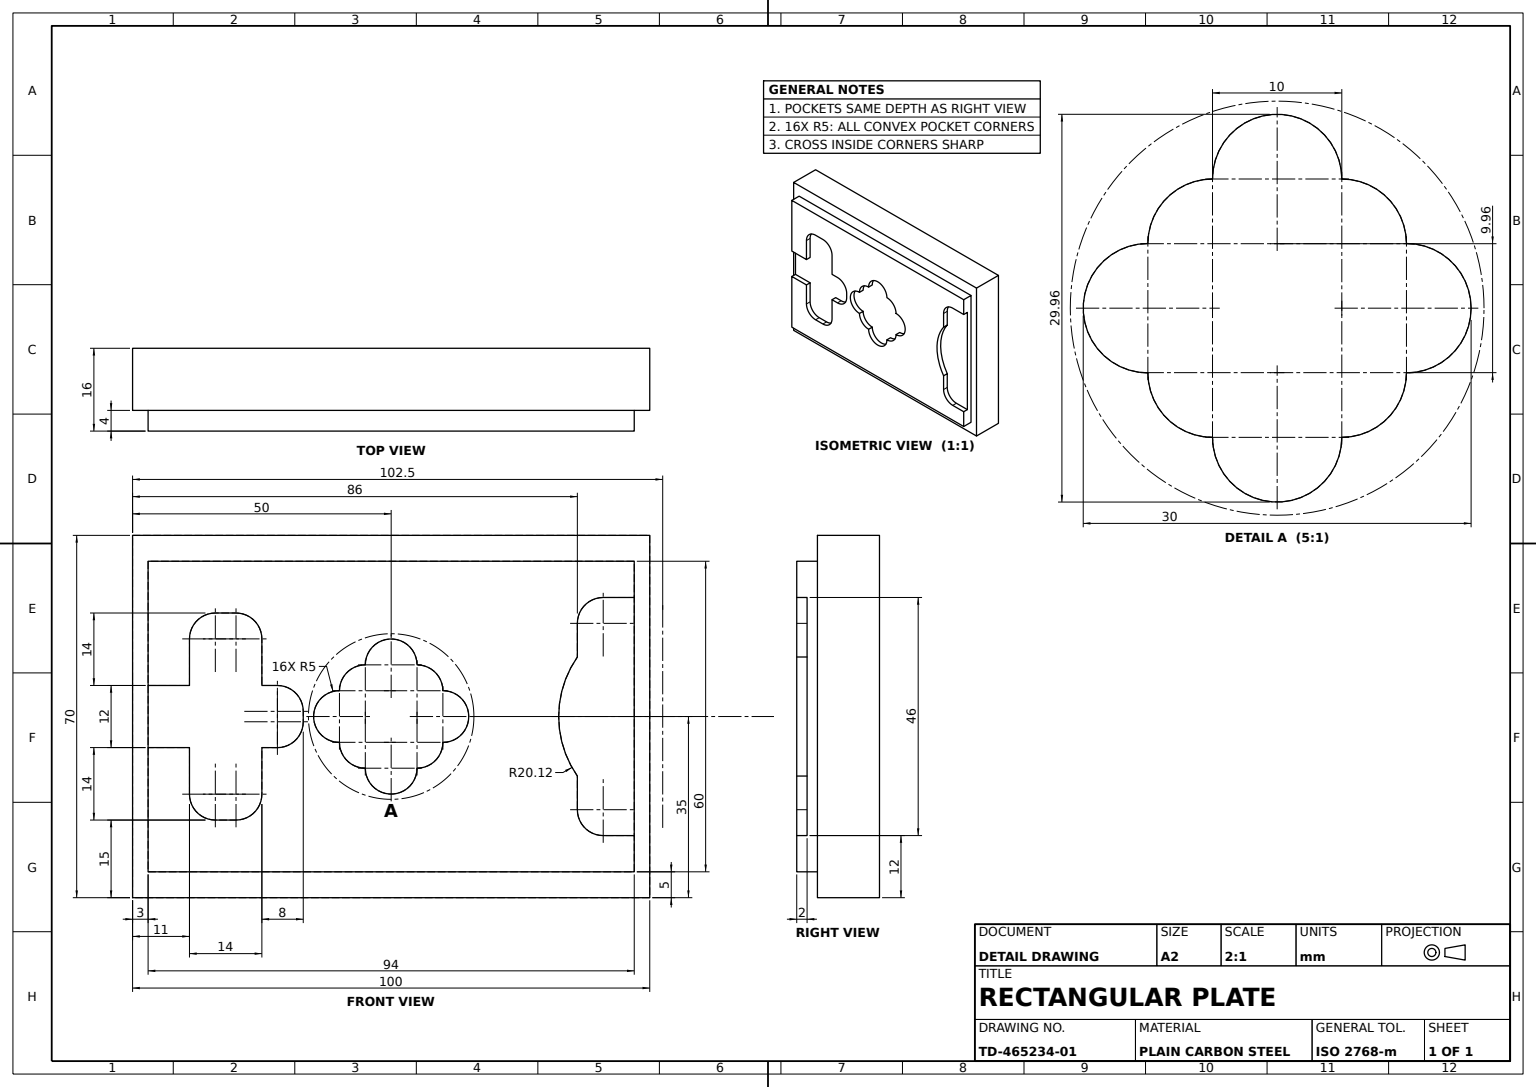
ISO-10303-21;
HEADER;
FILE_DESCRIPTION((''),'2;1');
FILE_NAME('','',(''),(''),'','','');
FILE_SCHEMA(('AUTOMOTIVE_DESIGN'));
ENDSEC;
DATA;
#1=APPLICATION_CONTEXT('');
#2=PRODUCT_CONTEXT('',#1,'mechanical');
#3=PRODUCT('','','',(#2));
#4=PRODUCT_DEFINITION_FORMATION('','',#3);
#5=PRODUCT_DEFINITION_CONTEXT('',#1,'design');
#6=PRODUCT_DEFINITION('','',#4,#5);
#7=PRODUCT_DEFINITION_SHAPE('','',#6);
#8=(LENGTH_UNIT()NAMED_UNIT(*)SI_UNIT(.MILLI.,.METRE.));
#9=(NAMED_UNIT(*)PLANE_ANGLE_UNIT()SI_UNIT($,.RADIAN.));
#10=(NAMED_UNIT(*)SI_UNIT($,.STERADIAN.)SOLID_ANGLE_UNIT());
#11=UNCERTAINTY_MEASURE_WITH_UNIT(LENGTH_MEASURE(1.E-05),#8,'distance_accuracy_value','');
#12=(GEOMETRIC_REPRESENTATION_CONTEXT(3)GLOBAL_UNCERTAINTY_ASSIGNED_CONTEXT((#11))GLOBAL_UNIT_ASSIGNED_CONTEXT((#8,#9,#10))REPRESENTATION_CONTEXT('',''));
#13=CARTESIAN_POINT('',(17.,-1.010637,-10.));
#14=VERTEX_POINT('',#13);
#15=CARTESIAN_POINT('',(17.,1.,-10.));
#16=VERTEX_POINT('',#15);
#17=CARTESIAN_POINT('',(17.,0.,-10.));
#18=DIRECTION('',(0.,1.,0.));
#19=VECTOR('',#18,1000.);
#20=LINE('',#17,#19);
#21=EDGE_CURVE('',#14,#16,#20,.T.);
#22=ORIENTED_EDGE('',*,*,#21,.T.);
#23=CARTESIAN_POINT('',(17.,1.,-8.));
#24=VERTEX_POINT('',#23);
#25=DIRECTION('',(0.,0.,-1.));
#26=VECTOR('',#25,1000.);
#27=LINE('',#23,#26);
#28=EDGE_CURVE('',#24,#16,#27,.T.);
#29=ORIENTED_EDGE('',*,*,#28,.F.);
#30=CARTESIAN_POINT('',(17.,-1.010637,-8.));
#31=VERTEX_POINT('',#30);
#32=DIRECTION('',(0.,-1.,0.));
#33=VECTOR('',#32,1000.);
#34=LINE('',#23,#33);
#35=EDGE_CURVE('',#24,#31,#34,.T.);
#36=ORIENTED_EDGE('',*,*,#35,.T.);
#37=LINE('',#30,#26);
#38=EDGE_CURVE('',#31,#14,#37,.T.);
#39=ORIENTED_EDGE('',*,*,#38,.T.);
#40=EDGE_LOOP('',(#22,#29,#36,#39));
#41=FACE_OUTER_BOUND('',#40,.T.);
#42=DIRECTION('',(1.,0.,0.));
#43=AXIS2_PLACEMENT_3D('',#23,#42,#25);
#44=PLANE('',#43);
#45=ADVANCED_FACE('',(#41),#44,.T.);
#46=CARTESIAN_POINT('',(47.,-30.,-6.));
#47=VERTEX_POINT('',#46);
#48=CARTESIAN_POINT('',(-47.,-30.,-6.));
#49=VERTEX_POINT('',#48);
#50=DIRECTION('',(-1.,0.,0.));
#51=VECTOR('',#50,1000.);
#52=LINE('',#48,#51);
#53=EDGE_CURVE('',#47,#49,#52,.T.);
#54=ORIENTED_EDGE('',*,*,#53,.F.);
#55=CARTESIAN_POINT('',(47.,30.,-6.));
#56=VERTEX_POINT('',#55);
#57=LINE('',#55,#33);
#58=EDGE_CURVE('',#56,#47,#57,.T.);
#59=ORIENTED_EDGE('',*,*,#58,.F.);
#60=CARTESIAN_POINT('',(-47.,30.,-6.));
#61=VERTEX_POINT('',#60);
#62=VECTOR('',#42,1000.);
#63=LINE('',#60,#62);
#64=EDGE_CURVE('',#61,#56,#63,.T.);
#65=ORIENTED_EDGE('',*,*,#64,.F.);
#66=LINE('',#60,#19);
#67=EDGE_CURVE('',#49,#61,#66,.T.);
#68=ORIENTED_EDGE('',*,*,#67,.F.);
#69=EDGE_LOOP('',(#54,#59,#65,#68));
#70=FACE_BOUND('',#69,.T.);
#71=CARTESIAN_POINT('',(-50.,-35.,-6.));
#72=VERTEX_POINT('',#71);
#73=CARTESIAN_POINT('',(50.,-35.,-6.));
#74=VERTEX_POINT('',#73);
#75=LINE('',#71,#62);
#76=EDGE_CURVE('',#72,#74,#75,.T.);
#77=ORIENTED_EDGE('',*,*,#76,.F.);
#78=CARTESIAN_POINT('',(-50.,35.,-6.));
#79=VERTEX_POINT('',#78);
#80=LINE('',#78,#33);
#81=EDGE_CURVE('',#79,#72,#80,.T.);
#82=ORIENTED_EDGE('',*,*,#81,.F.);
#83=CARTESIAN_POINT('',(50.,35.,-6.));
#84=VERTEX_POINT('',#83);
#85=LINE('',#78,#51);
#86=EDGE_CURVE('',#84,#79,#85,.T.);
#87=ORIENTED_EDGE('',*,*,#86,.F.);
#88=LINE('',#83,#19);
#89=EDGE_CURVE('',#74,#84,#88,.T.);
#90=ORIENTED_EDGE('',*,*,#89,.F.);
#91=EDGE_LOOP('',(#77,#82,#87,#90));
#92=FACE_OUTER_BOUND('',#91,.T.);
#93=CARTESIAN_POINT('',(0.,0.,-6.));
#94=DIRECTION('',(0.,0.,1.));
#95=AXIS2_PLACEMENT_3D('',#93,#94,#42);
#96=PLANE('',#95);
#97=ADVANCED_FACE('',(#70,#92),#96,.F.);
#98=CARTESIAN_POINT('',(-50.,35.,6.));
#99=VERTEX_POINT('',#98);
#100=CARTESIAN_POINT('',(-50.,-35.,6.));
#101=VERTEX_POINT('',#100);
#102=LINE('',#98,#33);
#103=EDGE_CURVE('',#99,#101,#102,.T.);
#104=ORIENTED_EDGE('',*,*,#103,.F.);
#105=LINE('',#98,#26);
#106=EDGE_CURVE('',#99,#79,#105,.T.);
#107=ORIENTED_EDGE('',*,*,#106,.T.);
#108=ORIENTED_EDGE('',*,*,#81,.T.);
#109=LINE('',#100,#26);
#110=EDGE_CURVE('',#101,#72,#109,.T.);
#111=ORIENTED_EDGE('',*,*,#110,.F.);
#112=EDGE_LOOP('',(#104,#107,#108,#111));
#113=FACE_OUTER_BOUND('',#112,.T.);
#114=AXIS2_PLACEMENT_3D('',#98,#42,#18);
#115=PLANE('',#114);
#116=ADVANCED_FACE('',(#113),#115,.F.);
#117=CARTESIAN_POINT('',(5.000015,9.982432,-8.));
#118=VERTEX_POINT('',#117);
#119=CARTESIAN_POINT('',(5.000015,9.982432,-10.));
#120=VERTEX_POINT('',#119);
#121=LINE('',#117,#26);
#122=EDGE_CURVE('',#118,#120,#121,.T.);
#123=ORIENTED_EDGE('',*,*,#122,.T.);
#124=CARTESIAN_POINT('',(10.,5.000015,-10.));
#125=VERTEX_POINT('',#124);
#126=CARTESIAN_POINT('',(5.000015,4.982416,-10.));
#127=AXIS2_PLACEMENT_3D('',#126,#25,#42);
#128=CIRCLE('',#127,5.000015);
#129=EDGE_CURVE('',#120,#125,#128,.T.);
#130=ORIENTED_EDGE('',*,*,#129,.T.);
#131=CARTESIAN_POINT('',(10.,5.000015,-8.));
#132=VERTEX_POINT('',#131);
#133=LINE('',#131,#26);
#134=EDGE_CURVE('',#132,#125,#133,.T.);
#135=ORIENTED_EDGE('',*,*,#134,.F.);
#136=CARTESIAN_POINT('',(5.000015,4.982416,-8.));
#137=AXIS2_PLACEMENT_3D('',#136,#94,#42);
#138=CIRCLE('',#137,5.000015);
#139=EDGE_CURVE('',#132,#118,#138,.T.);
#140=ORIENTED_EDGE('',*,*,#139,.T.);
#141=EDGE_LOOP('',(#123,#130,#135,#140));
#142=FACE_OUTER_BOUND('',#141,.T.);
#143=AXIS2_PLACEMENT_3D('',#136,#25,#50);
#144=CYLINDRICAL_SURFACE('',#143,5.000015);
#145=ADVANCED_FACE('',(#142),#144,.F.);
#146=ORIENTED_EDGE('',*,*,#89,.T.);
#147=CARTESIAN_POINT('',(50.,35.,6.));
#148=VERTEX_POINT('',#147);
#149=LINE('',#147,#26);
#150=EDGE_CURVE('',#148,#84,#149,.T.);
#151=ORIENTED_EDGE('',*,*,#150,.F.);
#152=CARTESIAN_POINT('',(50.,-35.,6.));
#153=VERTEX_POINT('',#152);
#154=LINE('',#147,#19);
#155=EDGE_CURVE('',#153,#148,#154,.T.);
#156=ORIENTED_EDGE('',*,*,#155,.F.);
#157=LINE('',#152,#26);
#158=EDGE_CURVE('',#153,#74,#157,.T.);
#159=ORIENTED_EDGE('',*,*,#158,.T.);
#160=EDGE_LOOP('',(#146,#151,#156,#159));
#161=FACE_OUTER_BOUND('',#160,.T.);
#162=AXIS2_PLACEMENT_3D('',#147,#50,#94);
#163=PLANE('',#162);
#164=ADVANCED_FACE('',(#161),#163,.F.);
#165=CARTESIAN_POINT('',(-47.,-30.,-10.));
#166=VERTEX_POINT('',#165);
#167=VECTOR('',#94,1000.);
#168=LINE('',#165,#167);
#169=EDGE_CURVE('',#166,#49,#168,.T.);
#170=ORIENTED_EDGE('',*,*,#169,.F.);
#171=CARTESIAN_POINT('',(47.,-30.,-10.));
#172=VERTEX_POINT('',#171);
#173=LINE('',#165,#51);
#174=EDGE_CURVE('',#172,#166,#173,.T.);
#175=ORIENTED_EDGE('',*,*,#174,.F.);
#176=LINE('',#171,#167);
#177=EDGE_CURVE('',#172,#47,#176,.T.);
#178=ORIENTED_EDGE('',*,*,#177,.T.);
#179=ORIENTED_EDGE('',*,*,#53,.T.);
#180=EDGE_LOOP('',(#170,#175,#178,#179));
#181=FACE_OUTER_BOUND('',#180,.T.);
#182=AXIS2_PLACEMENT_3D('',#165,#18,#50);
#183=PLANE('',#182);
#184=ADVANCED_FACE('',(#181),#183,.F.);
#185=CARTESIAN_POINT('',(-36.,11.5,-10.));
#186=VERTEX_POINT('',#185);
#187=CARTESIAN_POINT('',(-36.,18.,-10.));
#188=VERTEX_POINT('',#187);
#189=CARTESIAN_POINT('',(-36.,0.,-10.));
#190=LINE('',#189,#19);
#191=EDGE_CURVE('',#186,#188,#190,.T.);
#192=ORIENTED_EDGE('',*,*,#191,.F.);
#193=CARTESIAN_POINT('',(-36.,11.5,-8.));
#194=VERTEX_POINT('',#193);
#195=LINE('',#193,#26);
#196=EDGE_CURVE('',#194,#186,#195,.T.);
#197=ORIENTED_EDGE('',*,*,#196,.F.);
#198=CARTESIAN_POINT('',(-36.,18.,-8.));
#199=VERTEX_POINT('',#198);
#200=LINE('',#198,#33);
#201=EDGE_CURVE('',#199,#194,#200,.T.);
#202=ORIENTED_EDGE('',*,*,#201,.F.);
#203=LINE('',#198,#26);
#204=EDGE_CURVE('',#199,#188,#203,.T.);
#205=ORIENTED_EDGE('',*,*,#204,.T.);
#206=EDGE_LOOP('',(#192,#197,#202,#205));
#207=FACE_OUTER_BOUND('',#206,.T.);
#208=AXIS2_PLACEMENT_3D('',#198,#42,#25);
#209=PLANE('',#208);
#210=ADVANCED_FACE('',(#207),#209,.F.);
#211=CARTESIAN_POINT('',(-5.000015,-9.982432,-8.));
#212=VERTEX_POINT('',#211);
#213=CARTESIAN_POINT('',(-5.000015,-9.982432,-10.));
#214=VERTEX_POINT('',#213);
#215=LINE('',#211,#26);
#216=EDGE_CURVE('',#212,#214,#215,.T.);
#217=ORIENTED_EDGE('',*,*,#216,.T.);
#218=CARTESIAN_POINT('',(-10.,-5.000015,-10.));
#219=VERTEX_POINT('',#218);
#220=CARTESIAN_POINT('',(-5.000015,-4.982416,-10.));
#221=AXIS2_PLACEMENT_3D('',#220,#25,#42);
#222=CIRCLE('',#221,5.000015);
#223=EDGE_CURVE('',#214,#219,#222,.T.);
#224=ORIENTED_EDGE('',*,*,#223,.T.);
#225=CARTESIAN_POINT('',(-10.,-5.000015,-8.));
#226=VERTEX_POINT('',#225);
#227=LINE('',#225,#26);
#228=EDGE_CURVE('',#226,#219,#227,.T.);
#229=ORIENTED_EDGE('',*,*,#228,.F.);
#230=CARTESIAN_POINT('',(-5.000015,-4.982416,-8.));
#231=AXIS2_PLACEMENT_3D('',#230,#94,#42);
#232=CIRCLE('',#231,5.000015);
#233=EDGE_CURVE('',#226,#212,#232,.T.);
#234=ORIENTED_EDGE('',*,*,#233,.T.);
#235=EDGE_LOOP('',(#217,#224,#229,#234));
#236=FACE_OUTER_BOUND('',#235,.T.);
#237=AXIS2_PLACEMENT_3D('',#230,#25,#50);
#238=CYLINDRICAL_SURFACE('',#237,5.000015);
#239=ADVANCED_FACE('',(#236),#238,.F.);
#240=CARTESIAN_POINT('',(25.,6.,-10.));
#241=VERTEX_POINT('',#240);
#242=CARTESIAN_POINT('',(25.,15.,-10.));
#243=VERTEX_POINT('',#242);
#244=CARTESIAN_POINT('',(25.,0.,-10.));
#245=LINE('',#244,#19);
#246=EDGE_CURVE('',#241,#243,#245,.T.);
#247=ORIENTED_EDGE('',*,*,#246,.T.);
#248=CARTESIAN_POINT('',(25.,15.,-8.));
#249=VERTEX_POINT('',#248);
#250=LINE('',#248,#26);
#251=EDGE_CURVE('',#249,#243,#250,.T.);
#252=ORIENTED_EDGE('',*,*,#251,.F.);
#253=CARTESIAN_POINT('',(25.,6.,-8.));
#254=VERTEX_POINT('',#253);
#255=LINE('',#248,#33);
#256=EDGE_CURVE('',#249,#254,#255,.T.);
#257=ORIENTED_EDGE('',*,*,#256,.T.);
#258=LINE('',#253,#26);
#259=EDGE_CURVE('',#254,#241,#258,.T.);
#260=ORIENTED_EDGE('',*,*,#259,.T.);
#261=EDGE_LOOP('',(#247,#252,#257,#260));
#262=FACE_OUTER_BOUND('',#261,.T.);
#263=AXIS2_PLACEMENT_3D('',#248,#42,#25);
#264=PLANE('',#263);
#265=ADVANCED_FACE('',(#262),#264,.T.);
#266=CARTESIAN_POINT('',(22.,6.,-8.));
#267=VERTEX_POINT('',#266);
#268=CARTESIAN_POINT('',(22.,6.,-10.));
#269=VERTEX_POINT('',#268);
#270=LINE('',#266,#26);
#271=EDGE_CURVE('',#267,#269,#270,.T.);
#272=ORIENTED_EDGE('',*,*,#271,.T.);
#273=CARTESIAN_POINT('',(0.,6.,-10.));
#274=LINE('',#273,#62);
#275=EDGE_CURVE('',#269,#241,#274,.T.);
#276=ORIENTED_EDGE('',*,*,#275,.T.);
#277=ORIENTED_EDGE('',*,*,#259,.F.);
#278=LINE('',#253,#51);
#279=EDGE_CURVE('',#254,#267,#278,.T.);
#280=ORIENTED_EDGE('',*,*,#279,.T.);
#281=EDGE_LOOP('',(#272,#276,#277,#280));
#282=FACE_OUTER_BOUND('',#281,.T.);
#283=AXIS2_PLACEMENT_3D('',#253,#32,#25);
#284=PLANE('',#283);
#285=ADVANCED_FACE('',(#282),#284,.T.);
#286=CARTESIAN_POINT('',(22.017781,-6.010605,-10.));
#287=VERTEX_POINT('',#286);
#288=CARTESIAN_POINT('',(22.,-1.010637,-10.));
#289=AXIS2_PLACEMENT_3D('',#288,#25,#42);
#290=CIRCLE('',#289,5.);
#291=EDGE_CURVE('',#287,#14,#290,.T.);
#292=ORIENTED_EDGE('',*,*,#291,.T.);
#293=ORIENTED_EDGE('',*,*,#38,.F.);
#294=CARTESIAN_POINT('',(22.017781,-6.010605,-8.));
#295=VERTEX_POINT('',#294);
#296=CARTESIAN_POINT('',(22.,-1.010637,-8.));
#297=AXIS2_PLACEMENT_3D('',#296,#94,#42);
#298=CIRCLE('',#297,5.);
#299=EDGE_CURVE('',#31,#295,#298,.T.);
#300=ORIENTED_EDGE('',*,*,#299,.T.);
#301=LINE('',#294,#26);
#302=EDGE_CURVE('',#295,#287,#301,.T.);
#303=ORIENTED_EDGE('',*,*,#302,.T.);
#304=EDGE_LOOP('',(#292,#293,#300,#303));
#305=FACE_OUTER_BOUND('',#304,.T.);
#306=AXIS2_PLACEMENT_3D('',#296,#25,#50);
#307=CYLINDRICAL_SURFACE('',#306,5.);
#308=ADVANCED_FACE('',(#305),#307,.F.);
#309=CARTESIAN_POINT('',(-41.,-23.,-10.));
#310=VERTEX_POINT('',#309);
#311=CARTESIAN_POINT('',(-47.,-23.,-10.));
#312=VERTEX_POINT('',#311);
#313=CARTESIAN_POINT('',(0.,-23.,-10.));
#314=LINE('',#313,#51);
#315=EDGE_CURVE('',#310,#312,#314,.T.);
#316=ORIENTED_EDGE('',*,*,#315,.F.);
#317=CARTESIAN_POINT('',(-36.,-18.,-10.));
#318=VERTEX_POINT('',#317);
#319=CARTESIAN_POINT('',(-41.,-18.,-10.));
#320=AXIS2_PLACEMENT_3D('',#319,#25,#42);
#321=CIRCLE('',#320,5.);
#322=EDGE_CURVE('',#318,#310,#321,.T.);
#323=ORIENTED_EDGE('',*,*,#322,.F.);
#324=CARTESIAN_POINT('',(-36.,-11.5,-10.));
#325=VERTEX_POINT('',#324);
#326=LINE('',#189,#33);
#327=EDGE_CURVE('',#325,#318,#326,.T.);
#328=ORIENTED_EDGE('',*,*,#327,.F.);
#329=CARTESIAN_POINT('',(-52.504998,0.,-10.));
#330=AXIS2_PLACEMENT_3D('',#329,#25,#42);
#331=CIRCLE('',#330,20.116286);
#332=EDGE_CURVE('',#186,#325,#331,.T.);
#333=ORIENTED_EDGE('',*,*,#332,.F.);
#334=ORIENTED_EDGE('',*,*,#191,.T.);
#335=CARTESIAN_POINT('',(-41.,23.,-10.));
#336=VERTEX_POINT('',#335);
#337=CARTESIAN_POINT('',(-41.,18.,-10.));
#338=AXIS2_PLACEMENT_3D('',#337,#94,#42);
#339=CIRCLE('',#338,5.);
#340=EDGE_CURVE('',#188,#336,#339,.T.);
#341=ORIENTED_EDGE('',*,*,#340,.T.);
#342=CARTESIAN_POINT('',(-47.,23.,-10.));
#343=VERTEX_POINT('',#342);
#344=CARTESIAN_POINT('',(0.,23.,-10.));
#345=LINE('',#344,#51);
#346=EDGE_CURVE('',#336,#343,#345,.T.);
#347=ORIENTED_EDGE('',*,*,#346,.T.);
#348=CARTESIAN_POINT('',(-47.,30.,-10.));
#349=VERTEX_POINT('',#348);
#350=LINE('',#348,#19);
#351=EDGE_CURVE('',#343,#349,#350,.T.);
#352=ORIENTED_EDGE('',*,*,#351,.T.);
#353=CARTESIAN_POINT('',(47.,30.,-10.));
#354=VERTEX_POINT('',#353);
#355=LINE('',#348,#62);
#356=EDGE_CURVE('',#349,#354,#355,.T.);
#357=ORIENTED_EDGE('',*,*,#356,.T.);
#358=CARTESIAN_POINT('',(47.,6.,-10.));
#359=VERTEX_POINT('',#358);
#360=LINE('',#353,#33);
#361=EDGE_CURVE('',#354,#359,#360,.T.);
#362=ORIENTED_EDGE('',*,*,#361,.T.);
#363=CARTESIAN_POINT('',(39.,6.,-10.));
#364=VERTEX_POINT('',#363);
#365=EDGE_CURVE('',#364,#359,#274,.T.);
#366=ORIENTED_EDGE('',*,*,#365,.F.);
#367=CARTESIAN_POINT('',(39.,15.,-10.));
#368=VERTEX_POINT('',#367);
#369=CARTESIAN_POINT('',(39.,0.,-10.));
#370=LINE('',#369,#19);
#371=EDGE_CURVE('',#364,#368,#370,.T.);
#372=ORIENTED_EDGE('',*,*,#371,.T.);
#373=CARTESIAN_POINT('',(34.,20.,-10.));
#374=VERTEX_POINT('',#373);
#375=CARTESIAN_POINT('',(34.,15.,-10.));
#376=AXIS2_PLACEMENT_3D('',#375,#94,#42);
#377=CIRCLE('',#376,5.);
#378=EDGE_CURVE('',#368,#374,#377,.T.);
#379=ORIENTED_EDGE('',*,*,#378,.T.);
#380=CARTESIAN_POINT('',(30.,20.,-10.));
#381=VERTEX_POINT('',#380);
#382=CARTESIAN_POINT('',(0.,20.,-10.));
#383=LINE('',#382,#62);
#384=EDGE_CURVE('',#381,#374,#383,.T.);
#385=ORIENTED_EDGE('',*,*,#384,.F.);
#386=CARTESIAN_POINT('',(30.,15.,-10.));
#387=AXIS2_PLACEMENT_3D('',#386,#25,#42);
#388=CIRCLE('',#387,5.);
#389=EDGE_CURVE('',#243,#381,#388,.T.);
#390=ORIENTED_EDGE('',*,*,#389,.F.);
#391=ORIENTED_EDGE('',*,*,#246,.F.);
#392=ORIENTED_EDGE('',*,*,#275,.F.);
#393=CARTESIAN_POINT('',(22.,1.,-10.));
#394=AXIS2_PLACEMENT_3D('',#393,#94,#42);
#395=CIRCLE('',#394,5.);
#396=EDGE_CURVE('',#269,#16,#395,.T.);
#397=ORIENTED_EDGE('',*,*,#396,.T.);
#398=ORIENTED_EDGE('',*,*,#21,.F.);
#399=ORIENTED_EDGE('',*,*,#291,.F.);
#400=CARTESIAN_POINT('',(25.,-6.,-10.));
#401=VERTEX_POINT('',#400);
#402=CARTESIAN_POINT('',(0.021653,-6.088828,-10.));
#403=DIRECTION('',(-0.999993677,-0.003556172,0.));
#404=VECTOR('',#403,1000.);
#405=LINE('',#402,#404);
#406=EDGE_CURVE('',#401,#287,#405,.T.);
#407=ORIENTED_EDGE('',*,*,#406,.F.);
#408=CARTESIAN_POINT('',(25.,-15.,-10.));
#409=VERTEX_POINT('',#408);
#410=LINE('',#244,#33);
#411=EDGE_CURVE('',#401,#409,#410,.T.);
#412=ORIENTED_EDGE('',*,*,#411,.T.);
#413=CARTESIAN_POINT('',(30.,-20.,-10.));
#414=VERTEX_POINT('',#413);
#415=CARTESIAN_POINT('',(30.,-15.,-10.));
#416=AXIS2_PLACEMENT_3D('',#415,#94,#42);
#417=CIRCLE('',#416,5.);
#418=EDGE_CURVE('',#409,#414,#417,.T.);
#419=ORIENTED_EDGE('',*,*,#418,.T.);
#420=CARTESIAN_POINT('',(34.,-20.,-10.));
#421=VERTEX_POINT('',#420);
#422=CARTESIAN_POINT('',(0.,-20.,-10.));
#423=LINE('',#422,#62);
#424=EDGE_CURVE('',#414,#421,#423,.T.);
#425=ORIENTED_EDGE('',*,*,#424,.T.);
#426=CARTESIAN_POINT('',(39.,-15.,-10.));
#427=VERTEX_POINT('',#426);
#428=CARTESIAN_POINT('',(34.,-15.,-10.));
#429=AXIS2_PLACEMENT_3D('',#428,#25,#42);
#430=CIRCLE('',#429,5.);
#431=EDGE_CURVE('',#427,#421,#430,.T.);
#432=ORIENTED_EDGE('',*,*,#431,.F.);
#433=CARTESIAN_POINT('',(39.,-6.,-10.));
#434=VERTEX_POINT('',#433);
#435=EDGE_CURVE('',#427,#434,#370,.T.);
#436=ORIENTED_EDGE('',*,*,#435,.T.);
#437=CARTESIAN_POINT('',(47.,-6.,-10.));
#438=VERTEX_POINT('',#437);
#439=CARTESIAN_POINT('',(0.,-6.,-10.));
#440=LINE('',#439,#62);
#441=EDGE_CURVE('',#434,#438,#440,.T.);
#442=ORIENTED_EDGE('',*,*,#441,.T.);
#443=EDGE_CURVE('',#438,#172,#360,.T.);
#444=ORIENTED_EDGE('',*,*,#443,.T.);
#445=ORIENTED_EDGE('',*,*,#174,.T.);
#446=EDGE_CURVE('',#166,#312,#350,.T.);
#447=ORIENTED_EDGE('',*,*,#446,.T.);
#448=EDGE_LOOP('',(#316,#323,#328,#333,#334,#341,#347,#352,#357,#362,#366,#372,#379,#385,#390,#391,#392,#397,#398,#399,#407,#412,#419,#425,#432,#436,#442,#444,#445,#447));
#449=FACE_OUTER_BOUND('',#448,.T.);
#450=CARTESIAN_POINT('',(-5.000015,9.982432,-10.));
#451=VERTEX_POINT('',#450);
#452=CARTESIAN_POINT('',(0.,9.982432,-10.));
#453=AXIS2_PLACEMENT_3D('',#452,#94,#42);
#454=CIRCLE('',#453,5.000015);
#455=EDGE_CURVE('',#120,#451,#454,.T.);
#456=ORIENTED_EDGE('',*,*,#455,.T.);
#457=CARTESIAN_POINT('',(-10.,5.000015,-10.));
#458=VERTEX_POINT('',#457);
#459=CARTESIAN_POINT('',(-5.000015,4.982416,-10.));
#460=AXIS2_PLACEMENT_3D('',#459,#94,#42);
#461=CIRCLE('',#460,5.000015);
#462=EDGE_CURVE('',#451,#458,#461,.T.);
#463=ORIENTED_EDGE('',*,*,#462,.T.);
#464=CARTESIAN_POINT('',(-15.000015,0.,-10.));
#465=VERTEX_POINT('',#464);
#466=CARTESIAN_POINT('',(-10.,0.,-10.));
#467=AXIS2_PLACEMENT_3D('',#466,#94,#42);
#468=CIRCLE('',#467,5.000015);
#469=EDGE_CURVE('',#458,#465,#468,.T.);
#470=ORIENTED_EDGE('',*,*,#469,.T.);
#471=EDGE_CURVE('',#465,#219,#468,.T.);
#472=ORIENTED_EDGE('',*,*,#471,.T.);
#473=ORIENTED_EDGE('',*,*,#223,.F.);
#474=CARTESIAN_POINT('',(5.000015,-9.982432,-10.));
#475=VERTEX_POINT('',#474);
#476=CARTESIAN_POINT('',(0.,-9.982432,-10.));
#477=AXIS2_PLACEMENT_3D('',#476,#94,#42);
#478=CIRCLE('',#477,5.000015);
#479=EDGE_CURVE('',#214,#475,#478,.T.);
#480=ORIENTED_EDGE('',*,*,#479,.T.);
#481=CARTESIAN_POINT('',(10.,-5.000015,-10.));
#482=VERTEX_POINT('',#481);
#483=CARTESIAN_POINT('',(5.000015,-4.982416,-10.));
#484=AXIS2_PLACEMENT_3D('',#483,#94,#42);
#485=CIRCLE('',#484,5.000015);
#486=EDGE_CURVE('',#475,#482,#485,.T.);
#487=ORIENTED_EDGE('',*,*,#486,.T.);
#488=CARTESIAN_POINT('',(10.,0.,-10.));
#489=AXIS2_PLACEMENT_3D('',#488,#94,#42);
#490=CIRCLE('',#489,5.000015);
#491=EDGE_CURVE('',#482,#125,#490,.T.);
#492=ORIENTED_EDGE('',*,*,#491,.T.);
#493=ORIENTED_EDGE('',*,*,#129,.F.);
#494=EDGE_LOOP('',(#456,#463,#470,#472,#473,#480,#487,#492,#493));
#495=FACE_BOUND('',#494,.T.);
#496=CARTESIAN_POINT('',(0.,0.,-10.));
#497=AXIS2_PLACEMENT_3D('',#496,#94,#42);
#498=PLANE('',#497);
#499=ADVANCED_FACE('',(#449,#495),#498,.F.);
#500=ORIENTED_EDGE('',*,*,#406,.T.);
#501=ORIENTED_EDGE('',*,*,#302,.F.);
#502=CARTESIAN_POINT('',(25.,-6.,-8.));
#503=VERTEX_POINT('',#502);
#504=DIRECTION('',(0.999993677,0.003556172,0.));
#505=VECTOR('',#504,1000.);
#506=LINE('',#294,#505);
#507=EDGE_CURVE('',#295,#503,#506,.T.);
#508=ORIENTED_EDGE('',*,*,#507,.T.);
#509=LINE('',#502,#26);
#510=EDGE_CURVE('',#503,#401,#509,.T.);
#511=ORIENTED_EDGE('',*,*,#510,.T.);
#512=EDGE_LOOP('',(#500,#501,#508,#511));
#513=FACE_OUTER_BOUND('',#512,.T.);
#514=DIRECTION('',(-0.003556172,0.999993677,0.));
#515=AXIS2_PLACEMENT_3D('',#294,#514,#403);
#516=PLANE('',#515);
#517=ADVANCED_FACE('',(#513),#516,.T.);
#518=ORIENTED_EDGE('',*,*,#389,.T.);
#519=CARTESIAN_POINT('',(30.,20.,-8.));
#520=VERTEX_POINT('',#519);
#521=LINE('',#519,#26);
#522=EDGE_CURVE('',#520,#381,#521,.T.);
#523=ORIENTED_EDGE('',*,*,#522,.F.);
#524=CARTESIAN_POINT('',(30.,15.,-8.));
#525=AXIS2_PLACEMENT_3D('',#524,#94,#42);
#526=CIRCLE('',#525,5.);
#527=EDGE_CURVE('',#520,#249,#526,.T.);
#528=ORIENTED_EDGE('',*,*,#527,.T.);
#529=ORIENTED_EDGE('',*,*,#251,.T.);
#530=EDGE_LOOP('',(#518,#523,#528,#529));
#531=FACE_OUTER_BOUND('',#530,.T.);
#532=AXIS2_PLACEMENT_3D('',#524,#25,#50);
#533=CYLINDRICAL_SURFACE('',#532,5.);
#534=ADVANCED_FACE('',(#531),#533,.F.);
#535=CARTESIAN_POINT('',(-36.,-18.,-8.));
#536=VERTEX_POINT('',#535);
#537=LINE('',#535,#26);
#538=EDGE_CURVE('',#536,#318,#537,.T.);
#539=ORIENTED_EDGE('',*,*,#538,.F.);
#540=CARTESIAN_POINT('',(-36.,-11.5,-8.));
#541=VERTEX_POINT('',#540);
#542=LINE('',#535,#19);
#543=EDGE_CURVE('',#536,#541,#542,.T.);
#544=ORIENTED_EDGE('',*,*,#543,.T.);
#545=LINE('',#540,#26);
#546=EDGE_CURVE('',#541,#325,#545,.T.);
#547=ORIENTED_EDGE('',*,*,#546,.T.);
#548=ORIENTED_EDGE('',*,*,#327,.T.);
#549=EDGE_LOOP('',(#539,#544,#547,#548));
#550=FACE_OUTER_BOUND('',#549,.T.);
#551=AXIS2_PLACEMENT_3D('',#535,#50,#94);
#552=PLANE('',#551);
#553=ADVANCED_FACE('',(#550),#552,.T.);
#554=CARTESIAN_POINT('',(-47.,-23.,-8.));
#555=VERTEX_POINT('',#554);
#556=LINE('',#554,#26);
#557=EDGE_CURVE('',#555,#312,#556,.T.);
#558=ORIENTED_EDGE('',*,*,#557,.F.);
#559=CARTESIAN_POINT('',(-41.,-23.,-8.));
#560=VERTEX_POINT('',#559);
#561=LINE('',#554,#62);
#562=EDGE_CURVE('',#555,#560,#561,.T.);
#563=ORIENTED_EDGE('',*,*,#562,.T.);
#564=LINE('',#559,#26);
#565=EDGE_CURVE('',#560,#310,#564,.T.);
#566=ORIENTED_EDGE('',*,*,#565,.T.);
#567=ORIENTED_EDGE('',*,*,#315,.T.);
#568=EDGE_LOOP('',(#558,#563,#566,#567));
#569=FACE_OUTER_BOUND('',#568,.T.);
#570=AXIS2_PLACEMENT_3D('',#554,#18,#94);
#571=PLANE('',#570);
#572=ADVANCED_FACE('',(#569),#571,.T.);
#573=CARTESIAN_POINT('',(10.,-5.000015,-8.));
#574=VERTEX_POINT('',#573);
#575=CARTESIAN_POINT('',(5.000015,-9.982432,-8.));
#576=VERTEX_POINT('',#575);
#577=CARTESIAN_POINT('',(5.000015,-4.982416,-8.));
#578=AXIS2_PLACEMENT_3D('',#577,#25,#50);
#579=CIRCLE('',#578,5.000015);
#580=EDGE_CURVE('',#574,#576,#579,.T.);
#581=ORIENTED_EDGE('',*,*,#580,.T.);
#582=CARTESIAN_POINT('',(0.,-9.982432,-8.));
#583=AXIS2_PLACEMENT_3D('',#582,#25,#50);
#584=CIRCLE('',#583,5.000015);
#585=EDGE_CURVE('',#576,#212,#584,.T.);
#586=ORIENTED_EDGE('',*,*,#585,.T.);
#587=ORIENTED_EDGE('',*,*,#233,.F.);
#588=CARTESIAN_POINT('',(-15.000015,0.,-8.));
#589=VERTEX_POINT('',#588);
#590=CARTESIAN_POINT('',(-10.,0.,-8.));
#591=AXIS2_PLACEMENT_3D('',#590,#25,#50);
#592=CIRCLE('',#591,5.000015);
#593=EDGE_CURVE('',#226,#589,#592,.T.);
#594=ORIENTED_EDGE('',*,*,#593,.T.);
#595=CARTESIAN_POINT('',(-10.,5.000015,-8.));
#596=VERTEX_POINT('',#595);
#597=EDGE_CURVE('',#589,#596,#592,.T.);
#598=ORIENTED_EDGE('',*,*,#597,.T.);
#599=CARTESIAN_POINT('',(-5.000015,9.982432,-8.));
#600=VERTEX_POINT('',#599);
#601=CARTESIAN_POINT('',(-5.000015,4.982416,-8.));
#602=AXIS2_PLACEMENT_3D('',#601,#25,#50);
#603=CIRCLE('',#602,5.000015);
#604=EDGE_CURVE('',#596,#600,#603,.T.);
#605=ORIENTED_EDGE('',*,*,#604,.T.);
#606=CARTESIAN_POINT('',(0.,9.982432,-8.));
#607=AXIS2_PLACEMENT_3D('',#606,#25,#50);
#608=CIRCLE('',#607,5.000015);
#609=EDGE_CURVE('',#600,#118,#608,.T.);
#610=ORIENTED_EDGE('',*,*,#609,.T.);
#611=ORIENTED_EDGE('',*,*,#139,.F.);
#612=CARTESIAN_POINT('',(10.,0.,-8.));
#613=AXIS2_PLACEMENT_3D('',#612,#25,#50);
#614=CIRCLE('',#613,5.000015);
#615=EDGE_CURVE('',#132,#574,#614,.T.);
#616=ORIENTED_EDGE('',*,*,#615,.T.);
#617=EDGE_LOOP('',(#581,#586,#587,#594,#598,#605,#610,#611,#616));
#618=FACE_OUTER_BOUND('',#617,.T.);
#619=CARTESIAN_POINT('',(2.500008,7.482424,-8.));
#620=AXIS2_PLACEMENT_3D('',#619,#94,#42);
#621=PLANE('',#620);
#622=ADVANCED_FACE('',(#618),#621,.F.);
#623=CARTESIAN_POINT('',(47.,6.,-8.));
#624=VERTEX_POINT('',#623);
#625=CARTESIAN_POINT('',(39.,6.,-8.));
#626=VERTEX_POINT('',#625);
#627=LINE('',#623,#51);
#628=EDGE_CURVE('',#624,#626,#627,.T.);
#629=ORIENTED_EDGE('',*,*,#628,.T.);
#630=LINE('',#625,#26);
#631=EDGE_CURVE('',#626,#364,#630,.T.);
#632=ORIENTED_EDGE('',*,*,#631,.T.);
#633=ORIENTED_EDGE('',*,*,#365,.T.);
#634=LINE('',#623,#26);
#635=EDGE_CURVE('',#624,#359,#634,.T.);
#636=ORIENTED_EDGE('',*,*,#635,.F.);
#637=EDGE_LOOP('',(#629,#632,#633,#636));
#638=FACE_OUTER_BOUND('',#637,.T.);
#639=AXIS2_PLACEMENT_3D('',#623,#32,#25);
#640=PLANE('',#639);
#641=ADVANCED_FACE('',(#638),#640,.T.);
#642=CARTESIAN_POINT('',(34.,-20.,-8.));
#643=VERTEX_POINT('',#642);
#644=CARTESIAN_POINT('',(30.,-20.,-8.));
#645=VERTEX_POINT('',#644);
#646=LINE('',#642,#51);
#647=EDGE_CURVE('',#643,#645,#646,.T.);
#648=ORIENTED_EDGE('',*,*,#647,.F.);
#649=LINE('',#642,#26);
#650=EDGE_CURVE('',#643,#421,#649,.T.);
#651=ORIENTED_EDGE('',*,*,#650,.T.);
#652=ORIENTED_EDGE('',*,*,#424,.F.);
#653=LINE('',#644,#26);
#654=EDGE_CURVE('',#645,#414,#653,.T.);
#655=ORIENTED_EDGE('',*,*,#654,.F.);
#656=EDGE_LOOP('',(#648,#651,#652,#655));
#657=FACE_OUTER_BOUND('',#656,.T.);
#658=AXIS2_PLACEMENT_3D('',#642,#32,#25);
#659=PLANE('',#658);
#660=ADVANCED_FACE('',(#657),#659,.F.);
#661=CARTESIAN_POINT('',(-47.,23.,-8.));
#662=VERTEX_POINT('',#661);
#663=CARTESIAN_POINT('',(-41.,23.,-8.));
#664=VERTEX_POINT('',#663);
#665=LINE('',#661,#62);
#666=EDGE_CURVE('',#662,#664,#665,.T.);
#667=ORIENTED_EDGE('',*,*,#666,.F.);
#668=LINE('',#661,#26);
#669=EDGE_CURVE('',#662,#343,#668,.T.);
#670=ORIENTED_EDGE('',*,*,#669,.T.);
#671=ORIENTED_EDGE('',*,*,#346,.F.);
#672=LINE('',#663,#26);
#673=EDGE_CURVE('',#664,#336,#672,.T.);
#674=ORIENTED_EDGE('',*,*,#673,.F.);
#675=EDGE_LOOP('',(#667,#670,#671,#674));
#676=FACE_OUTER_BOUND('',#675,.T.);
#677=AXIS2_PLACEMENT_3D('',#661,#18,#94);
#678=PLANE('',#677);
#679=ADVANCED_FACE('',(#676),#678,.F.);
#680=ORIENTED_EDGE('',*,*,#122,.F.);
#681=ORIENTED_EDGE('',*,*,#609,.F.);
#682=LINE('',#599,#26);
#683=EDGE_CURVE('',#600,#451,#682,.T.);
#684=ORIENTED_EDGE('',*,*,#683,.T.);
#685=ORIENTED_EDGE('',*,*,#455,.F.);
#686=EDGE_LOOP('',(#680,#681,#684,#685));
#687=FACE_OUTER_BOUND('',#686,.T.);
#688=CYLINDRICAL_SURFACE('',#607,5.000015);
#689=ADVANCED_FACE('',(#687),#688,.F.);
#690=ORIENTED_EDGE('',*,*,#110,.T.);
#691=ORIENTED_EDGE('',*,*,#76,.T.);
#692=ORIENTED_EDGE('',*,*,#158,.F.);
#693=LINE('',#100,#62);
#694=EDGE_CURVE('',#101,#153,#693,.T.);
#695=ORIENTED_EDGE('',*,*,#694,.F.);
#696=EDGE_LOOP('',(#690,#691,#692,#695));
#697=FACE_OUTER_BOUND('',#696,.T.);
#698=AXIS2_PLACEMENT_3D('',#100,#18,#94);
#699=PLANE('',#698);
#700=ADVANCED_FACE('',(#697),#699,.F.);
#701=CARTESIAN_POINT('',(25.,-15.,-8.));
#702=VERTEX_POINT('',#701);
#703=LINE('',#701,#19);
#704=EDGE_CURVE('',#702,#503,#703,.T.);
#705=ORIENTED_EDGE('',*,*,#704,.F.);
#706=LINE('',#701,#26);
#707=EDGE_CURVE('',#702,#409,#706,.T.);
#708=ORIENTED_EDGE('',*,*,#707,.T.);
#709=ORIENTED_EDGE('',*,*,#411,.F.);
#710=ORIENTED_EDGE('',*,*,#510,.F.);
#711=EDGE_LOOP('',(#705,#708,#709,#710));
#712=FACE_OUTER_BOUND('',#711,.T.);
#713=AXIS2_PLACEMENT_3D('',#701,#50,#94);
#714=PLANE('',#713);
#715=ADVANCED_FACE('',(#712),#714,.F.);
#716=ORIENTED_EDGE('',*,*,#628,.F.);
#717=CARTESIAN_POINT('',(47.,-6.,-8.));
#718=VERTEX_POINT('',#717);
#719=LINE('',#717,#19);
#720=EDGE_CURVE('',#718,#624,#719,.T.);
#721=ORIENTED_EDGE('',*,*,#720,.F.);
#722=CARTESIAN_POINT('',(39.,-6.,-8.));
#723=VERTEX_POINT('',#722);
#724=LINE('',#717,#51);
#725=EDGE_CURVE('',#718,#723,#724,.T.);
#726=ORIENTED_EDGE('',*,*,#725,.T.);
#727=CARTESIAN_POINT('',(39.,-15.,-8.));
#728=VERTEX_POINT('',#727);
#729=LINE('',#722,#33);
#730=EDGE_CURVE('',#723,#728,#729,.T.);
#731=ORIENTED_EDGE('',*,*,#730,.T.);
#732=CARTESIAN_POINT('',(34.,-15.,-8.));
#733=AXIS2_PLACEMENT_3D('',#732,#94,#42);
#734=CIRCLE('',#733,5.);
#735=EDGE_CURVE('',#643,#728,#734,.T.);
#736=ORIENTED_EDGE('',*,*,#735,.F.);
#737=ORIENTED_EDGE('',*,*,#647,.T.);
#738=CARTESIAN_POINT('',(30.,-15.,-8.));
#739=AXIS2_PLACEMENT_3D('',#738,#25,#50);
#740=CIRCLE('',#739,5.);
#741=EDGE_CURVE('',#645,#702,#740,.T.);
#742=ORIENTED_EDGE('',*,*,#741,.T.);
#743=ORIENTED_EDGE('',*,*,#704,.T.);
#744=ORIENTED_EDGE('',*,*,#507,.F.);
#745=ORIENTED_EDGE('',*,*,#299,.F.);
#746=ORIENTED_EDGE('',*,*,#35,.F.);
#747=CARTESIAN_POINT('',(22.,1.,-8.));
#748=AXIS2_PLACEMENT_3D('',#747,#25,#50);
#749=CIRCLE('',#748,5.);
#750=EDGE_CURVE('',#24,#267,#749,.T.);
#751=ORIENTED_EDGE('',*,*,#750,.T.);
#752=ORIENTED_EDGE('',*,*,#279,.F.);
#753=ORIENTED_EDGE('',*,*,#256,.F.);
#754=ORIENTED_EDGE('',*,*,#527,.F.);
#755=CARTESIAN_POINT('',(34.,20.,-8.));
#756=VERTEX_POINT('',#755);
#757=LINE('',#755,#51);
#758=EDGE_CURVE('',#756,#520,#757,.T.);
#759=ORIENTED_EDGE('',*,*,#758,.F.);
#760=CARTESIAN_POINT('',(39.,15.,-8.));
#761=VERTEX_POINT('',#760);
#762=CARTESIAN_POINT('',(34.,15.,-8.));
#763=AXIS2_PLACEMENT_3D('',#762,#25,#50);
#764=CIRCLE('',#763,5.);
#765=EDGE_CURVE('',#756,#761,#764,.T.);
#766=ORIENTED_EDGE('',*,*,#765,.T.);
#767=LINE('',#760,#33);
#768=EDGE_CURVE('',#761,#626,#767,.T.);
#769=ORIENTED_EDGE('',*,*,#768,.T.);
#770=EDGE_LOOP('',(#716,#721,#726,#731,#736,#737,#742,#743,#744,#745,#746,#751,#752,#753,#754,#759,#766,#769));
#771=FACE_OUTER_BOUND('',#770,.T.);
#772=PLANE('',#525);
#773=ADVANCED_FACE('',(#771),#772,.F.);
#774=LINE('',#98,#51);
#775=EDGE_CURVE('',#148,#99,#774,.T.);
#776=ORIENTED_EDGE('',*,*,#775,.T.);
#777=ORIENTED_EDGE('',*,*,#103,.T.);
#778=ORIENTED_EDGE('',*,*,#694,.T.);
#779=ORIENTED_EDGE('',*,*,#155,.T.);
#780=EDGE_LOOP('',(#776,#777,#778,#779));
#781=FACE_OUTER_BOUND('',#780,.T.);
#782=CARTESIAN_POINT('',(0.,0.,6.));
#783=AXIS2_PLACEMENT_3D('',#782,#94,#42);
#784=PLANE('',#783);
#785=ADVANCED_FACE('',(#781),#784,.T.);
#786=ORIENTED_EDGE('',*,*,#543,.F.);
#787=CARTESIAN_POINT('',(-41.,-18.,-8.));
#788=AXIS2_PLACEMENT_3D('',#787,#94,#42);
#789=CIRCLE('',#788,5.);
#790=EDGE_CURVE('',#560,#536,#789,.T.);
#791=ORIENTED_EDGE('',*,*,#790,.F.);
#792=ORIENTED_EDGE('',*,*,#562,.F.);
#793=LINE('',#554,#19);
#794=EDGE_CURVE('',#555,#662,#793,.T.);
#795=ORIENTED_EDGE('',*,*,#794,.T.);
#796=ORIENTED_EDGE('',*,*,#666,.T.);
#797=CARTESIAN_POINT('',(-41.,18.,-8.));
#798=AXIS2_PLACEMENT_3D('',#797,#25,#50);
#799=CIRCLE('',#798,5.);
#800=EDGE_CURVE('',#664,#199,#799,.T.);
#801=ORIENTED_EDGE('',*,*,#800,.T.);
#802=ORIENTED_EDGE('',*,*,#201,.T.);
#803=CARTESIAN_POINT('',(-52.504998,0.,-8.));
#804=AXIS2_PLACEMENT_3D('',#803,#94,#42);
#805=CIRCLE('',#804,20.116286);
#806=EDGE_CURVE('',#541,#194,#805,.T.);
#807=ORIENTED_EDGE('',*,*,#806,.F.);
#808=EDGE_LOOP('',(#786,#791,#792,#795,#796,#801,#802,#807));
#809=FACE_OUTER_BOUND('',#808,.T.);
#810=PLANE('',#798);
#811=ADVANCED_FACE('',(#809),#810,.T.);
#812=ORIENTED_EDGE('',*,*,#725,.F.);
#813=LINE('',#717,#26);
#814=EDGE_CURVE('',#718,#438,#813,.T.);
#815=ORIENTED_EDGE('',*,*,#814,.T.);
#816=ORIENTED_EDGE('',*,*,#441,.F.);
#817=LINE('',#722,#26);
#818=EDGE_CURVE('',#723,#434,#817,.T.);
#819=ORIENTED_EDGE('',*,*,#818,.F.);
#820=EDGE_LOOP('',(#812,#815,#816,#819));
#821=FACE_OUTER_BOUND('',#820,.T.);
#822=AXIS2_PLACEMENT_3D('',#717,#32,#25);
#823=PLANE('',#822);
#824=ADVANCED_FACE('',(#821),#823,.F.);
#825=ORIENTED_EDGE('',*,*,#775,.F.);
#826=ORIENTED_EDGE('',*,*,#150,.T.);
#827=ORIENTED_EDGE('',*,*,#86,.T.);
#828=ORIENTED_EDGE('',*,*,#106,.F.);
#829=EDGE_LOOP('',(#825,#826,#827,#828));
#830=FACE_OUTER_BOUND('',#829,.T.);
#831=AXIS2_PLACEMENT_3D('',#98,#32,#25);
#832=PLANE('',#831);
#833=ADVANCED_FACE('',(#830),#832,.F.);
#834=ORIENTED_EDGE('',*,*,#479,.F.);
#835=ORIENTED_EDGE('',*,*,#216,.F.);
#836=ORIENTED_EDGE('',*,*,#585,.F.);
#837=LINE('',#575,#26);
#838=EDGE_CURVE('',#576,#475,#837,.T.);
#839=ORIENTED_EDGE('',*,*,#838,.T.);
#840=EDGE_LOOP('',(#834,#835,#836,#839));
#841=FACE_OUTER_BOUND('',#840,.T.);
#842=CYLINDRICAL_SURFACE('',#583,5.000015);
#843=ADVANCED_FACE('',(#841),#842,.F.);
#844=ORIENTED_EDGE('',*,*,#806,.T.);
#845=ORIENTED_EDGE('',*,*,#196,.T.);
#846=ORIENTED_EDGE('',*,*,#332,.T.);
#847=ORIENTED_EDGE('',*,*,#546,.F.);
#848=EDGE_LOOP('',(#844,#845,#846,#847));
#849=FACE_OUTER_BOUND('',#848,.T.);
#850=AXIS2_PLACEMENT_3D('',#803,#25,#50);
#851=CYLINDRICAL_SURFACE('',#850,20.116286);
#852=ADVANCED_FACE('',(#849),#851,.F.);
#853=LINE('',#595,#26);
#854=EDGE_CURVE('',#596,#458,#853,.T.);
#855=ORIENTED_EDGE('',*,*,#854,.F.);
#856=ORIENTED_EDGE('',*,*,#597,.F.);
#857=LINE('',#588,#26);
#858=EDGE_CURVE('',#589,#465,#857,.T.);
#859=ORIENTED_EDGE('',*,*,#858,.T.);
#860=ORIENTED_EDGE('',*,*,#469,.F.);
#861=EDGE_LOOP('',(#855,#856,#859,#860));
#862=FACE_OUTER_BOUND('',#861,.T.);
#863=CYLINDRICAL_SURFACE('',#591,5.000015);
#864=ADVANCED_FACE('',(#862),#863,.F.);
#865=LINE('',#348,#167);
#866=EDGE_CURVE('',#349,#61,#865,.T.);
#867=ORIENTED_EDGE('',*,*,#866,.T.);
#868=ORIENTED_EDGE('',*,*,#64,.T.);
#869=LINE('',#353,#167);
#870=EDGE_CURVE('',#354,#56,#869,.T.);
#871=ORIENTED_EDGE('',*,*,#870,.F.);
#872=ORIENTED_EDGE('',*,*,#356,.F.);
#873=EDGE_LOOP('',(#867,#868,#871,#872));
#874=FACE_OUTER_BOUND('',#873,.T.);
#875=AXIS2_PLACEMENT_3D('',#348,#32,#42);
#876=PLANE('',#875);
#877=ADVANCED_FACE('',(#874),#876,.F.);
#878=ORIENTED_EDGE('',*,*,#768,.F.);
#879=LINE('',#760,#26);
#880=EDGE_CURVE('',#761,#368,#879,.T.);
#881=ORIENTED_EDGE('',*,*,#880,.T.);
#882=ORIENTED_EDGE('',*,*,#371,.F.);
#883=ORIENTED_EDGE('',*,*,#631,.F.);
#884=EDGE_LOOP('',(#878,#881,#882,#883));
#885=FACE_OUTER_BOUND('',#884,.T.);
#886=AXIS2_PLACEMENT_3D('',#760,#42,#25);
#887=PLANE('',#886);
#888=ADVANCED_FACE('',(#885),#887,.F.);
#889=ORIENTED_EDGE('',*,*,#758,.T.);
#890=ORIENTED_EDGE('',*,*,#522,.T.);
#891=ORIENTED_EDGE('',*,*,#384,.T.);
#892=LINE('',#755,#26);
#893=EDGE_CURVE('',#756,#374,#892,.T.);
#894=ORIENTED_EDGE('',*,*,#893,.F.);
#895=EDGE_LOOP('',(#889,#890,#891,#894));
#896=FACE_OUTER_BOUND('',#895,.T.);
#897=AXIS2_PLACEMENT_3D('',#755,#32,#25);
#898=PLANE('',#897);
#899=ADVANCED_FACE('',(#896),#898,.T.);
#900=ORIENTED_EDGE('',*,*,#361,.F.);
#901=ORIENTED_EDGE('',*,*,#870,.T.);
#902=ORIENTED_EDGE('',*,*,#58,.T.);
#903=ORIENTED_EDGE('',*,*,#177,.F.);
#904=ORIENTED_EDGE('',*,*,#443,.F.);
#905=ORIENTED_EDGE('',*,*,#814,.F.);
#906=ORIENTED_EDGE('',*,*,#720,.T.);
#907=ORIENTED_EDGE('',*,*,#635,.T.);
#908=EDGE_LOOP('',(#900,#901,#902,#903,#904,#905,#906,#907));
#909=FACE_OUTER_BOUND('',#908,.T.);
#910=AXIS2_PLACEMENT_3D('',#353,#50,#32);
#911=PLANE('',#910);
#912=ADVANCED_FACE('',(#909),#911,.F.);
#913=ORIENTED_EDGE('',*,*,#340,.F.);
#914=ORIENTED_EDGE('',*,*,#204,.F.);
#915=ORIENTED_EDGE('',*,*,#800,.F.);
#916=ORIENTED_EDGE('',*,*,#673,.T.);
#917=EDGE_LOOP('',(#913,#914,#915,#916));
#918=FACE_OUTER_BOUND('',#917,.T.);
#919=CYLINDRICAL_SURFACE('',#798,5.);
#920=ADVANCED_FACE('',(#918),#919,.F.);
#921=ORIENTED_EDGE('',*,*,#741,.F.);
#922=ORIENTED_EDGE('',*,*,#654,.T.);
#923=ORIENTED_EDGE('',*,*,#418,.F.);
#924=ORIENTED_EDGE('',*,*,#707,.F.);
#925=EDGE_LOOP('',(#921,#922,#923,#924));
#926=FACE_OUTER_BOUND('',#925,.T.);
#927=CYLINDRICAL_SURFACE('',#739,5.);
#928=ADVANCED_FACE('',(#926),#927,.F.);
#929=ORIENTED_EDGE('',*,*,#683,.F.);
#930=ORIENTED_EDGE('',*,*,#604,.F.);
#931=ORIENTED_EDGE('',*,*,#854,.T.);
#932=ORIENTED_EDGE('',*,*,#462,.F.);
#933=EDGE_LOOP('',(#929,#930,#931,#932));
#934=FACE_OUTER_BOUND('',#933,.T.);
#935=CYLINDRICAL_SURFACE('',#602,5.000015);
#936=ADVANCED_FACE('',(#934),#935,.F.);
#937=LINE('',#573,#26);
#938=EDGE_CURVE('',#574,#482,#937,.T.);
#939=ORIENTED_EDGE('',*,*,#938,.F.);
#940=ORIENTED_EDGE('',*,*,#615,.F.);
#941=ORIENTED_EDGE('',*,*,#134,.T.);
#942=ORIENTED_EDGE('',*,*,#491,.F.);
#943=EDGE_LOOP('',(#939,#940,#941,#942));
#944=FACE_OUTER_BOUND('',#943,.T.);
#945=CYLINDRICAL_SURFACE('',#613,5.000015);
#946=ADVANCED_FACE('',(#944),#945,.F.);
#947=ORIENTED_EDGE('',*,*,#396,.F.);
#948=ORIENTED_EDGE('',*,*,#271,.F.);
#949=ORIENTED_EDGE('',*,*,#750,.F.);
#950=ORIENTED_EDGE('',*,*,#28,.T.);
#951=EDGE_LOOP('',(#947,#948,#949,#950));
#952=FACE_OUTER_BOUND('',#951,.T.);
#953=CYLINDRICAL_SURFACE('',#748,5.);
#954=ADVANCED_FACE('',(#952),#953,.F.);
#955=ORIENTED_EDGE('',*,*,#435,.F.);
#956=LINE('',#727,#26);
#957=EDGE_CURVE('',#728,#427,#956,.T.);
#958=ORIENTED_EDGE('',*,*,#957,.F.);
#959=ORIENTED_EDGE('',*,*,#730,.F.);
#960=ORIENTED_EDGE('',*,*,#818,.T.);
#961=EDGE_LOOP('',(#955,#958,#959,#960));
#962=FACE_OUTER_BOUND('',#961,.T.);
#963=AXIS2_PLACEMENT_3D('',#722,#42,#25);
#964=PLANE('',#963);
#965=ADVANCED_FACE('',(#962),#964,.F.);
#966=ORIENTED_EDGE('',*,*,#431,.T.);
#967=ORIENTED_EDGE('',*,*,#650,.F.);
#968=ORIENTED_EDGE('',*,*,#735,.T.);
#969=ORIENTED_EDGE('',*,*,#957,.T.);
#970=EDGE_LOOP('',(#966,#967,#968,#969));
#971=FACE_OUTER_BOUND('',#970,.T.);
#972=AXIS2_PLACEMENT_3D('',#732,#25,#50);
#973=CYLINDRICAL_SURFACE('',#972,5.);
#974=ADVANCED_FACE('',(#971),#973,.F.);
#975=ORIENTED_EDGE('',*,*,#880,.F.);
#976=ORIENTED_EDGE('',*,*,#765,.F.);
#977=ORIENTED_EDGE('',*,*,#893,.T.);
#978=ORIENTED_EDGE('',*,*,#378,.F.);
#979=EDGE_LOOP('',(#975,#976,#977,#978));
#980=FACE_OUTER_BOUND('',#979,.T.);
#981=CYLINDRICAL_SURFACE('',#763,5.);
#982=ADVANCED_FACE('',(#980),#981,.F.);
#983=ORIENTED_EDGE('',*,*,#486,.F.);
#984=ORIENTED_EDGE('',*,*,#838,.F.);
#985=ORIENTED_EDGE('',*,*,#580,.F.);
#986=ORIENTED_EDGE('',*,*,#938,.T.);
#987=EDGE_LOOP('',(#983,#984,#985,#986));
#988=FACE_OUTER_BOUND('',#987,.T.);
#989=CYLINDRICAL_SURFACE('',#578,5.000015);
#990=ADVANCED_FACE('',(#988),#989,.F.);
#991=ORIENTED_EDGE('',*,*,#322,.T.);
#992=ORIENTED_EDGE('',*,*,#565,.F.);
#993=ORIENTED_EDGE('',*,*,#790,.T.);
#994=ORIENTED_EDGE('',*,*,#538,.T.);
#995=EDGE_LOOP('',(#991,#992,#993,#994));
#996=FACE_OUTER_BOUND('',#995,.T.);
#997=AXIS2_PLACEMENT_3D('',#787,#25,#50);
#998=CYLINDRICAL_SURFACE('',#997,5.);
#999=ADVANCED_FACE('',(#996),#998,.F.);
#1000=ORIENTED_EDGE('',*,*,#593,.F.);
#1001=ORIENTED_EDGE('',*,*,#228,.T.);
#1002=ORIENTED_EDGE('',*,*,#471,.F.);
#1003=ORIENTED_EDGE('',*,*,#858,.F.);
#1004=EDGE_LOOP('',(#1000,#1001,#1002,#1003));
#1005=FACE_OUTER_BOUND('',#1004,.T.);
#1006=ADVANCED_FACE('',(#1005),#863,.F.);
#1007=ORIENTED_EDGE('',*,*,#669,.F.);
#1008=ORIENTED_EDGE('',*,*,#794,.F.);
#1009=ORIENTED_EDGE('',*,*,#557,.T.);
#1010=ORIENTED_EDGE('',*,*,#446,.F.);
#1011=ORIENTED_EDGE('',*,*,#169,.T.);
#1012=ORIENTED_EDGE('',*,*,#67,.T.);
#1013=ORIENTED_EDGE('',*,*,#866,.F.);
#1014=ORIENTED_EDGE('',*,*,#351,.F.);
#1015=EDGE_LOOP('',(#1007,#1008,#1009,#1010,#1011,#1012,#1013,#1014));
#1016=FACE_OUTER_BOUND('',#1015,.T.);
#1017=AXIS2_PLACEMENT_3D('',#348,#42,#18);
#1018=PLANE('',#1017);
#1019=ADVANCED_FACE('',(#1016),#1018,.F.);
#1020=CLOSED_SHELL('',(#45,#97,#116,#145,#164,#184,#210,#239,#265,#285,#308,#499,#517,#534,#553,#572,#622,#641,#660,#679,#689,#700,#715,#773,#785,#811,#824,#833,#843,#852,#864,#877,#888,#899,#912,#920,#928,#936,#946,#954,#965,#974,#982,#990,#999,#1006,#1019));
#1021=MANIFOLD_SOLID_BREP('',#1020);
#1022=ADVANCED_BREP_SHAPE_REPRESENTATION('',(#1021),#12);
#1023=SHAPE_DEFINITION_REPRESENTATION(#7,#1022);
ENDSEC;
END-ISO-10303-21;
